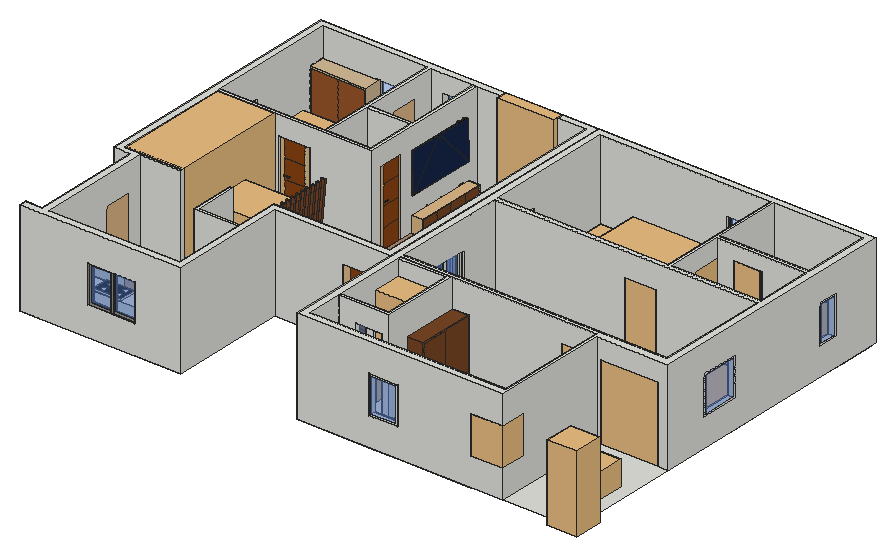
# SketchUp Ruby script. Lengths in inches.
U = 1.inch
M = Sketchup.active_model
def pt(a) = Geom::Point3d.new(a.map { |v| v * U })
def face(e, loops, mat)
  f = e.add_face(loops[0].map { |a| pt(a) })
  loops[1..].each { |l| e.add_face(l.map { |a| pt(a) }).erase! }
  f.material = f.back_material = mat if mat
  f
end
# faces: each face lists its corners as indices into pts; further lists are holes
def faces(e, pts, list, mat = nil) = list.each { |f| face(e, (f[0].is_a?(Array) ? f : [f]).map { |l| l.map { |i| pts[i] } }, mat) }
# xy, xz, yz: faces in a plane at the given z, y or x. An outline is a flat list of corners, or four numbers for a rectangle; further outlines are holes
def ring(l) = l.size == 4 ? [[l[0], l[1]], [l[2], l[1]], [l[2], l[3]], [l[0], l[3]]] : l.each_slice(2).to_a
def flat(e, list, mat, &to3) = list.each { |f| face(e, (f[0].is_a?(Array) ? f : [f]).map { |l| ring(l).map { |u, v| to3.(u, v) } }, mat) }
def xy(e, z, list, mat = nil) = flat(e, list, mat) { |x, y| [x, y, z] }
def xz(e, y, list, mat = nil) = flat(e, list, mat) { |x, z| [x, y, z] }
def yz(e, x, list, mat = nil) = flat(e, list, mat) { |y, z| [x, y, z] }
def lines(e, pts, list) = list.each { |a, b| e.add_line(pt(pts[a]), pt(pts[b])) }
# prism: a flat outline (further loops are holes) pulled along v
def prism(e, loops, v, mat = nil)
  f = face(e, loops, mat); d = Geom::Vector3d.new(v.map { |x| x * U })
  f.pushpull(f.normal.samedirection?(d) ? d.length : -d.length)
end
def box(e, o, s, mat = nil) = prism(e, [[o, [o[0] + s[0], o[1], o[2]], [o[0] + s[0], o[1] + s[1], o[2]], [o[0], o[1] + s[1], o[2]]]], [0, 0, s[2]], mat)
def at(x, y, z, deg = 0) = Geom::Transformation.translation(pt([x, y, z])) * Geom::Transformation.rotation(ORIGIN, Z_AXIS, deg.degrees)
def axes(o, x, y, z) = Geom::Transformation.new([*x, 0, *y, 0, *z, 0, *pt(o).to_a, 1])
def part(name) = M.definitions.add(name)
# library, detail: a bought-in or finely detailed component or shape, given as its bounding box
def library(name, o, s) = part(name).tap { |d| box(d.entities, o, s) }
def detail(e, o, s) = box(e.add_group.entities, o, s)
def put(e, d, t, mat = nil) = e.add_instance(d, t).tap { |i| i.material = mat if mat }
def group(e, t, mat = nil) = e.add_group.tap { |g| g.transformation = t; g.material = mat if mat }.entities
root = M.entities
M.materials.add("Sumele_Jewelry").color = [169, 169, 169]
M.materials.add("Walt_Disney_Pictures_intro_2006").color = [23, 39, 73]
M.materials.add("[0036_BurlyWood]").color = [222, 184, 135]
M.materials.add("[0042_Sienna]").color = [160, 82, 45]
M.materials.add("[0043_SaddleBrown]").color = [139, 69, 19]
M.materials.add("[0136_Charcoal]1").color = [35, 35, 35]
M.materials.add("[0137_Black]").color = [0, 0, 0]
M.materials.add("[Color M03]").color = [170, 170, 170]
M.materials.add("[Color M04]").color = [142, 142, 142]
M.materials.add("[Formica Beige]").color = [211, 187, 149]
M.materials.add("[Tile Veriegated Stone]").color = [171, 137, 112]
M.materials.add("[Translucent Glass Blue]").color = [100, 149, 237]
M.materials["[Translucent Glass Blue]"].alpha = 0.5
M.materials.add("[Wood Cherry Original]").color = [152, 86, 42]
M.materials.add("[Wood Veneer 01]").color = [120, 70, 37]
c1 = library("finestra due ante",[0,0,0],[4.72,47.24,55.51])
c2 = part("Janela aluminio")
xy(c2.entities,0,[[0,0,47.24,1.57],[23.62,1.57,47.24,2.76],[0,2.76,25.98,3.9375],[0,3.9375,47.24,5.91]])
xy(c2.entities,43.31,[[0,0,47.24,1.57],[23.62,1.57,47.24,2.76],[0,2.76,0,5.91,47.24,5.91,47.24,3.9375,25.98,3.9375,25.98,2.76],[25.98,2.76,47.24,3.9375]])
xz(c2.entities,1.57,[[0,0,23.62,0,23.62,41.34,21.26,41.34,21.26,1.97,1.97,1.97,1.97,41.34,23.62,41.34,23.62,43.31,0,43.31],[[23.62,0,47.24,43.31],[25.7,1.97,45.28,41.34]]])
xz(c2.entities,2.76,[[[0,0,23.62,43.31],[2.36,2.36,21.26,40.94]],[23.62,0,25.98,43.31]])
xz(c2.entities,2.76,[[2.36,2.36,21.26,40.94]],"[Translucent Glass Blue]")
xz(c2.entities,3.9375,[[25.98,0,25.98,2.36,44.88,2.36,44.88,40.94,25.98,40.94,25.98,43.31,47.24,43.31,47.24,0]])
xz(c2.entities,3.9375,[[25.98,2.36,44.88,40.94]],"[Translucent Glass Blue]")
yz(c2.entities,0,[[0,0,1.57,43.31],[2.76,0,5.91,43.31]])
yz(c2.entities,23.62,[[1.57,0,2.76,43.31]])
yz(c2.entities,25.98,[[2.76,0,3.9375,43.31]])
yz(c2.entities,47.24,[[0,0,1.57,43.31],[1.57,0,2.76,43.31],[3.9375,0,5.91,43.31]])
c3 = library("Dining Table",[-4.14,-4.14,0],[95.74,137.21,49.0625])
c4 = library("sofa2 (2)",[-0.48,-0.6,0],[71.59,32.48,33.44])
c5 = library("Sofa S1 (2)",[1.47,3.82,0],[91.78,124.8,36.68])
c6 = library("Спалня Венид",[0.07,-0.07,0],[84.71,86.8,39])
c7 = library("70s+Toilet",[-10,-32.21,0],[19.64,32.21,33.59])
c8 = library("60rd,27rd x30h",[0,0,0],[60,60,30.5])
c9 = library("Dressing Table",[-15.16,-2.63,-1.96],[42.78,16.8,62.56])
c10 = library("Shower area",[0,0,0],[40.02,56.82,78.19])
c11 = library("Object02",[-606.68,-655.71,-190.21],[1149.33,653.61,1636.06])
c12 = part("skp42")
put(c12.entities,c11,at(0,0,0))
c13 = part("Senza")
put(c13.entities,c12,at(-166.13,607.08,194.25))
c14 = library("porta 4",[0.2,-5.42,1.33],[46.55,4.72,83.21])
c15 = library("door58",[0,0,0],[34.0625,4.69,78.29])
c16 = library("Vented interior door",[-3.9375,-3.9375,0],[8.49,35.4375,80.68])
c17 = library("Table And Chair",[-36.07,-19.67,0],[55.74,39.34,31.28])
c18 = library("Maple - Red Upright",[-19.73,-16.92,0],[37.29,36.93,96.9])
c19 = library("steps",[5.95,0,1.76],[152,98,97.5])
c20 = library("Sans titre",[-0.34,-1.41,0],[30.55,15.68,32.3])
c21 = part("Group\#3")
xy(c21.entities,0,[[0,1,48,10]])
xy(c21.entities,44.2,[[35,10,46,12]],"[0137_Black]")
xy(c21.entities,45.2,[[35,10,46,12]],"[0137_Black]")
xy(c21.entities,48.93,[[7.7,0,16.7,1]],"[0137_Black]")
xy(c21.entities,49.93,[[7.7,0,16.7,1]],"[0137_Black]")
xy(c21.entities,89,[[0,1,48,10]],"[0036_BurlyWood]")
xz(c21.entities,0,[[7.7,48.93,16.7,49.93]],"[0137_Black]")
xz(c21.entities,1,[[0,0,9.13,0,9.13,48.93,7.7,48.93,7.7,49.93,9.13,49.93,9.13,89,0,89],[40.3,0,48,89]],"[0036_BurlyWood]")
xz(c21.entities,1,[[9.13,0,40.3,22.78],[9.13,22.78,40.3,45.5625],[9.13,45.5625,40.3,45.5625,40.3,68.35,9.13,68.35,9.13,49.93,16.7,49.93,16.7,48.93,9.13,48.93],[9.13,68.35,40.3,89]],"[0043_SaddleBrown]")
xz(c21.entities,10,[[[0,0,48,89],[35,44.2,46,45.2]]],"[0036_BurlyWood]")
xz(c21.entities,12,[[35,44.2,46,45.2]],"[0137_Black]")
yz(c21.entities,0,[[1,0,10,89]],"[0036_BurlyWood]")
yz(c21.entities,7.7,[[0,48.93,1,49.93]],"[0137_Black]")
yz(c21.entities,16.7,[[0,48.93,1,49.93]],"[0137_Black]")
yz(c21.entities,35,[[10,44.2,12,45.2]],"[0137_Black]")
yz(c21.entities,46,[[10,44.2,12,45.2]],"[0137_Black]")
yz(c21.entities,48,[[1,0,10,89]],"[0036_BurlyWood]")
c22 = library("Group\#41",[0,0,0],[50.5,52.39,66.5])
c23 = library("Group\#65",[-3.51,-3.3,0],[107.56,127.46,42.43])
c24 = library("Group\#64",[0,0,0.08],[17.41,128.86,87.4])
c25 = library("组\#105",[-65.55,-8.17,-53.72],[35.57,34.93,21.52])
c26 = library("组\#276",[0,0,0],[31.5,32.28,31.05])
xy(root,16.749,[[351,11.292,351,96.867,360,96.867,360,20.292,442.282,20.292,442.282,11.292],[442.282,11.292,478.282,20.292],[478.282,11.292,571.5,20.292],[571.5,15.792,571.5,20.292,607.5,20.292,607.5,44.292,612,44.292,612,15.792],[607.5,44.292,607.5,164.292,603,164.292,603,168.792,616.5,168.792,616.5,159.792,612,159.792,612,44.292],
  [351,96.867,360,120.818],[351,120.818,351,216.792,360,216.792,360,168.792,564,168.792,564,164.292,360,164.292,360,120.818],[688.5,159.792,688.5,168.792,693,168.792,693,216.792,702,216.792,702,159.792],[351,216.792,360,264.792],[693,216.792,702,264.792],
  [351,264.792,351,328.131,360,328.131,360,317.292,525,317.292,525,312.792,360,312.792,360,264.792],[693,264.792,693,312.792,564,312.792,564,317.292,576,317.292,576,353.292,580.5,353.292,580.5,317.292,693,317.292,693,389.292,634.5,389.292,634.5,393.792,693,393.792,693,400.358,702,400.358,702,264.792],[351,328.131,360,376.131],[351,376.131,351,488.292,520.31,488.292,520.31,479.292,360,479.292,360,376.131],[576,389.292,576,479.292,580.5,479.292,580.5,393.792,601.5,393.792,601.5,389.292],
  [693,400.358,702,424.319],[693,424.319,693,479.292,568.31,479.292,568.31,488.292,702,488.292,702,424.319],[520.31,479.292,568.31,488.292]])
xy(root,16.749,[[0,11.292,15.884,20.292],[[21.884,11.292,204,11.292,204,159.792,351,162.4375,351,488.292,21.884,488.292],[188.5,238.792,193,240.792],[188.5,230.792,193,232.792],[188.5,222.792,193,224.792],[188.5,214.792,193,216.792],[188.5,206.792,193,208.792],[188.5,198.792,193,200.792],[188.5,190.792,193,192.792],[188.5,182.792,193,184.792],[188.5,174.792,193,176.792]],[0,159.792,15.884,488.292]],"[Tile Veriegated Stone]")
xy(root,16.749,[[188.5,174.792,193,176.792],[188.5,182.792,193,184.792],[188.5,190.792,193,192.792],[188.5,198.792,193,200.792],[188.5,206.792,193,208.792],
  [188.5,214.792,193,216.792],[188.5,222.792,193,224.792],[188.5,230.792,193,232.792],[188.5,238.792,193,240.792]],"[Wood Veneer 01]")
xy(root,52.749,[[442.282,11.292,478.282,20.292],[571.5,11.292,612,11.292,612,44.292,607.5,44.292,607.5,20.292,571.5,20.292],[351,96.867,360,120.818],[351,216.792,360,264.792],[693,216.792,702,264.792],
  [351,328.131,360,376.131],[693,400.358,702,424.319],[520.31,479.292,568.31,488.292]])
xy(root,54.656,[[399.065,317.292,512.065,318.292]],"[0137_Black]")
xy(root,59.632,[[204,375.393,206,460.393]],"[0137_Black]")
xy(root,64.749,[[83.903,21.989,119.903,44.041]])
xy(root,64.923,[[140,441.855,141,449.855]],"[0137_Black]")
xy(root,66.749,[[93.688,24.547,94.474,24.65,95.205,24.95,95.834,25.428,96.316,26.051,96.619,26.776,96.722,27.554,96.619,28.333,96.316,29.058,95.834,29.681,95.205,30.158,94.474,30.459,93.688,30.561,92.903,30.459,92.171,30.158,91.543,29.681,91.061,29.058,90.758,28.333,90.654,27.554,90.758,26.776,91.061,26.051,91.543,25.428,92.171,24.95,92.903,24.65],[112.904,24.547,113.689,24.65,114.421,24.95,115.049,25.428,115.531,26.051,115.834,26.776,115.9375,27.554,115.834,28.333,115.531,29.058,115.049,29.681,114.421,30.158,113.689,30.459,112.904,30.561,112.118,30.459,111.387,30.158,110.758,29.681,110.276,29.058,109.973,28.333,109.87,27.554,109.973,26.776,110.276,26.051,110.758,25.428,111.387,24.95,112.118,24.65],[93.688,34.571,94.474,34.673,95.205,34.974,95.834,35.451,96.316,36.074,96.619,36.8,96.722,37.578,96.619,38.356,96.316,39.081,95.834,39.704,95.205,40.182,94.474,40.482,93.688,40.585,92.903,40.482,92.171,40.182,91.543,39.704,91.061,39.081,90.758,38.356,90.654,37.578,90.758,36.8,91.061,36.074,91.543,35.451,92.171,34.974,92.903,34.673],[112.904,34.571,113.689,34.673,114.421,34.974,115.049,35.451,115.531,36.074,115.834,36.8,115.9375,37.578,115.834,38.356,115.531,39.081,115.049,39.704,114.421,40.182,113.689,40.482,112.904,40.585,112.118,40.482,111.387,40.182,110.758,39.704,110.276,39.081,109.973,38.356,109.87,37.578,109.973,36.8,110.276,36.074,110.758,35.451,111.387,34.974,112.118,34.673]])
xy(root,66.749,[[[83.903,21.989,119.903,44.041],[112.904,34.571,112.118,34.673,111.387,34.974,110.758,35.451,110.276,36.074,109.973,36.8,109.87,37.578,109.973,38.356,110.276,39.081,110.758,39.704,111.387,40.182,112.118,40.482,112.904,40.585,113.689,40.482,114.421,40.182,115.049,39.704,115.531,39.081,115.834,38.356,115.9375,37.578,115.834,36.8,115.531,36.074,115.049,35.451,114.421,34.974,113.689,34.673],[93.688,34.571,92.903,34.673,92.171,34.974,91.543,35.451,91.061,36.074,90.758,36.8,90.654,37.578,90.758,38.356,91.061,39.081,91.543,39.704,92.171,40.182,92.903,40.482,93.688,40.585,94.474,40.482,95.205,40.182,95.834,39.704,96.316,39.081,96.619,38.356,96.722,37.578,96.619,36.8,96.316,36.074,95.834,35.451,95.205,34.974,94.474,34.673],[112.904,24.547,112.118,24.65,111.387,24.95,110.758,25.428,110.276,26.051,109.973,26.776,109.87,27.554,109.973,28.333,110.276,29.058,110.758,29.681,111.387,30.158,112.118,30.459,112.904,30.561,113.689,30.459,114.421,30.158,115.049,29.681,115.531,29.058,115.834,28.333,115.9375,27.554,115.834,26.776,115.531,26.051,115.049,25.428,114.421,24.95,113.689,24.65],[93.688,24.547,92.903,24.65,92.171,24.95,91.543,25.428,91.061,26.051,90.758,26.776,90.654,27.554,90.758,28.333,91.061,29.058,91.543,29.681,92.171,30.158,92.903,30.459,93.688,30.561,94.474,30.459,95.205,30.158,95.834,29.681,96.316,29.058,96.619,28.333,96.722,27.554,96.619,26.776,96.316,26.051,95.834,25.428,95.205,24.95,94.474,24.65]]],"[0137_Black]")
xy(root,66.923,[[140,441.855,141,449.855]],"[0137_Black]")
xy(root,70.854,[[145.5,420.773,146.5,427.773]],"[0137_Black]")
xy(root,72.854,[[145.5,420.773,146.5,427.773]],"[0137_Black]")
xy(root,100.749,[[442.282,11.292,478.282,20.292],[571.5,11.292,612,15.792],[571.5,15.792,571.5,20.292,607.5,20.292,607.5,44.292,612,44.292,612,15.792],[351,96.867,360,120.818],[351,216.792,360,264.792],
  [693,216.792,702,264.792],[351,328.131,360,376.131],[693,400.358,702,424.319],[520.31,479.292,568.31,488.292]])
xy(root,101.656,[[399.065,317.292,512.065,318.292]],"[0137_Black]")
xy(root,105.749,[[525,312.792,564,317.292]])
xy(root,109.749,[[564,164.292,603,168.792]])
xy(root,110.632,[[204,375.393,206,460.393]],"[0137_Black]")
xy(root,112.32,[[616.5,159.792,688.5,168.792]])
xy(root,112.749,[[576,353.292,580.5,389.292]])
xy(root,118.749,[[601.5,389.292,634.5,393.792]])
xy(root,136.749,[[[351,11.292,612,11.292,612,159.792,702,159.792,702,488.292,351,488.292],[360,168.792,693,312.792],[360,20.292,607.5,164.292],[360,317.292,576,479.292],[580.5,393.792,693,479.292],[580.5,317.292,693,389.292]]])
xy(root,136.749,[[199.5,174.792,204,176.792],[199.5,182.792,204,184.792],[199.5,190.792,204,192.792],[199.5,198.792,204,200.792],[199.5,206.792,204,208.792],
  [199.5,214.792,204,216.792],[199.5,222.792,204,224.792],[199.5,230.792,204,232.792],[199.5,238.792,204,240.792]],"[Wood Veneer 01]")
xz(root,11.292,[[[351,16.749,612,16.749,612,52.749,571.5,52.749,571.5,100.749,612,100.749,612,136.749,351,136.749],[442.282,52.749,478.282,100.749]],[[442.282,52.749,478.282,100.749],[444.461,54.927,476.103,98.57]]])
xz(root,11.292,[[444.461,54.927,476.103,98.57]],"[Translucent Glass Blue]")
xz(root,20.292,[[[360,16.749,360,136.749,607.5,136.749,607.5,100.749,571.5,100.749,571.5,52.749,607.5,52.749,607.5,16.749],[442.282,52.749,478.282,100.749]]])
xz(root,21.989,[[83.903,64.749,119.903,66.749]])
xz(root,44.041,[[83.903,64.749,119.903,66.749]])
xz(root,44.292,[[607.5,52.749,612,100.749]])
xz(root,96.867,[[351,52.749,360,100.749]])
xz(root,120.818,[[351,52.749,360,100.749]])
xz(root,159.792,[[612,16.749,616.5,16.749,616.5,112.32,688.5,112.32,688.5,16.749,702,16.749,702,136.749,612,136.749]])
xz(root,164.292,[[360,16.749,564,16.749,564,109.749,603,109.749,603,16.749,607.5,16.749,607.5,136.749,360,136.749]])
xz(root,168.792,[[360,16.749,360,136.749,693,136.749,693,16.749,688.5,16.749,688.5,112.32,616.5,112.32,616.5,16.749,603,16.749,603,109.749,564,109.749,564,16.749]])
xz(root,174.792,[[188.5,16.749,193,16.749,204,136.749,199.5,136.749]],"[Wood Veneer 01]")
xz(root,176.792,[[188.5,16.749,199.5,136.749,204,136.749,193,16.749]],"[Wood Veneer 01]")
xz(root,182.792,[[188.5,16.749,193,16.749,204,136.749,199.5,136.749]],"[Wood Veneer 01]")
xz(root,184.792,[[188.5,16.749,199.5,136.749,204,136.749,193,16.749]],"[Wood Veneer 01]")
xz(root,190.792,[[188.5,16.749,193,16.749,204,136.749,199.5,136.749]],"[Wood Veneer 01]")
xz(root,192.792,[[188.5,16.749,199.5,136.749,204,136.749,193,16.749]],"[Wood Veneer 01]")
xz(root,198.792,[[188.5,16.749,193,16.749,204,136.749,199.5,136.749]],"[Wood Veneer 01]")
xz(root,200.792,[[188.5,16.749,199.5,136.749,204,136.749,193,16.749]],"[Wood Veneer 01]")
xz(root,206.792,[[188.5,16.749,193,16.749,204,136.749,199.5,136.749]],"[Wood Veneer 01]")
xz(root,208.792,[[188.5,16.749,199.5,136.749,204,136.749,193,16.749]],"[Wood Veneer 01]")
xz(root,214.792,[[188.5,16.749,193,16.749,204,136.749,199.5,136.749]],"[Wood Veneer 01]")
xz(root,216.792,[[351,52.749,360,100.749],[693,52.749,702,100.749]])
xz(root,216.792,[[188.5,16.749,199.5,136.749,204,136.749,193,16.749]],"[Wood Veneer 01]")
xz(root,222.792,[[188.5,16.749,193,16.749,204,136.749,199.5,136.749]],"[Wood Veneer 01]")
xz(root,224.792,[[188.5,16.749,199.5,136.749,204,136.749,193,16.749]],"[Wood Veneer 01]")
xz(root,230.792,[[188.5,16.749,193,16.749,204,136.749,199.5,136.749]],"[Wood Veneer 01]")
xz(root,232.792,[[188.5,16.749,199.5,136.749,204,136.749,193,16.749]],"[Wood Veneer 01]")
xz(root,238.792,[[188.5,16.749,193,16.749,204,136.749,199.5,136.749]],"[Wood Veneer 01]")
xz(root,240.792,[[188.5,16.749,199.5,136.749,204,136.749,193,16.749]],"[Wood Veneer 01]")
xz(root,264.792,[[351,52.749,360,100.749],[693,52.749,702,100.749]])
xz(root,312.792,[[360,16.749,525,16.749,525,105.749,564,105.749,564,16.749,693,16.749,693,136.749,360,136.749]])
xz(root,317.292,[[[360,16.749,360,136.749,576,136.749,576,16.749,564,16.749,564,105.749,525,105.749,525,16.749],[399.065,54.656,512.065,101.656]],[580.5,16.749,693,136.749]])
xz(root,318.292,[[399.065,54.656,512.065,101.656]],"[0137_Black]")
xz(root,328.131,[[351,52.749,360,100.749]])
xz(root,353.292,[[576,16.749,580.5,112.749]])
xz(root,375.393,[[204,59.632,206,110.632]],"[0137_Black]")
xz(root,376.131,[[351,52.749,360,100.749]])
xz(root,389.292,[[576,16.749,601.5,16.749,601.5,118.749,634.5,118.749,634.5,16.749,693,16.749,693,136.749,580.5,136.749,580.5,112.749,576,112.749]])
xz(root,393.792,[[580.5,16.749,580.5,136.749,693,136.749,693,16.749,634.5,16.749,634.5,118.749,601.5,118.749,601.5,16.749]])
xz(root,400.358,[[693,52.749,702,100.749]])
xz(root,420.773,[[145.5,70.854,146.5,72.854]],"[0137_Black]")
xz(root,424.319,[[693,52.749,702,100.749]])
xz(root,427.773,[[145.5,70.854,146.5,72.854]],"[0137_Black]")
xz(root,441.855,[[140,64.923,141,66.923]],"[0137_Black]")
xz(root,449.855,[[140,64.923,141,66.923]],"[0137_Black]")
xz(root,460.393,[[204,59.632,206,110.632]],"[0137_Black]")
xz(root,479.292,[[[360,16.749,576,136.749],[520.31,52.749,568.31,100.749]],[580.5,16.749,693,136.749]])
xz(root,488.292,[[[351,16.749,702,136.749],[520.31,52.749,568.31,100.749]]])
xz(root,488.292,[[[160.596,84.749,184.557,114.749],[162.026,86.179,183.127,113.319]]],"[Color M04]")
xz(root,488.292,[[162.026,86.179,183.127,113.319]],"[Translucent Glass Blue]")
yz(root,83.903,[[21.989,64.749,44.041,66.749]])
yz(root,119.903,[[21.989,64.749,44.041,66.749]])
yz(root,140,[[441.855,64.923,449.855,66.923]],"[0137_Black]")
yz(root,141,[[441.855,64.923,449.855,66.923]])
yz(root,145.5,[[420.773,70.854,427.773,72.854]])
yz(root,146.5,[[420.773,70.854,427.773,72.854]],"[0137_Black]")
yz(root,204,[[375.393,59.632,460.393,110.632]])
yz(root,206,[[375.393,59.632,460.393,110.632]],"[0137_Black]")
yz(root,351,[[[11.292,16.749,488.292,136.749],[328.131,52.749,376.131,100.749],[216.792,52.749,264.792,100.749],[96.867,52.749,120.818,100.749]],[[96.867,52.749,120.818,100.749],[98.43,54.312,119.255,99.185]]])
yz(root,351,[[98.43,54.312,119.255,99.185]],"[Translucent Glass Blue]")
yz(root,360,[[[20.292,16.749,164.292,136.749],[96.867,52.749,120.818,100.749]],[[168.792,16.749,312.792,136.749],[216.792,52.749,264.792,100.749]],[[317.292,16.749,479.292,136.749],[328.131,52.749,376.131,100.749]]])
yz(root,399.065,[[317.292,54.656,318.292,101.656]],"[0137_Black]")
yz(root,442.282,[[11.292,52.749,20.292,100.749]])
yz(root,478.282,[[11.292,52.749,20.292,100.749]])
yz(root,512.065,[[317.292,54.656,318.292,101.656]])
yz(root,520.31,[[479.292,52.749,488.292,100.749]])
yz(root,525,[[312.792,16.749,317.292,105.749]])
yz(root,564,[[164.292,16.749,168.792,109.749],[312.792,16.749,317.292,105.749]])
yz(root,568.31,[[479.292,52.749,488.292,100.749]])
yz(root,571.5,[[11.292,52.749,20.292,100.749]])
yz(root,576,[[317.292,16.749,317.292,136.749,479.292,136.749,479.292,16.749,389.292,16.749,389.292,112.749,353.292,112.749,353.292,16.749]])
yz(root,580.5,[[317.292,16.749,353.292,16.749,353.292,112.749,389.292,112.749,389.292,136.749,317.292,136.749],[393.792,16.749,479.292,136.749]])
yz(root,601.5,[[389.292,16.749,393.792,118.749]])
yz(root,603,[[164.292,16.749,168.792,109.749]])
yz(root,607.5,[[20.292,16.749,20.292,52.749,44.292,52.749,44.292,100.749,20.292,100.749,20.292,136.749,164.292,136.749,164.292,16.749]])
yz(root,612,[[11.292,16.749,159.792,16.749,159.792,136.749,11.292,136.749,11.292,100.749,44.292,100.749,44.292,52.749,11.292,52.749]])
yz(root,616.5,[[159.792,16.749,168.792,112.32]])
yz(root,634.5,[[389.292,16.749,393.792,118.749]])
yz(root,688.5,[[159.792,16.749,168.792,112.32]])
yz(root,693,[[[168.792,16.749,312.792,136.749],[216.792,52.749,264.792,100.749]],[317.292,16.749,389.292,136.749],[[393.792,16.749,479.292,136.749],[400.358,52.749,424.319,100.749]]])
yz(root,702,[[[159.792,16.749,488.292,136.749],[216.792,52.749,264.792,100.749],[400.358,52.749,424.319,100.749]],[[216.792,52.749,264.792,100.749],[218.515,54.472,263.068,99.026]],[[400.358,52.749,424.319,100.749],[401.857,54.248,422.82,99.249]]])
yz(root,702,[[401.857,54.248,422.82,99.249],[218.515,54.472,263.068,99.026]],"[Translucent Glass Blue]")
p = [[188.5,176.792,16.749],[188.5,174.792,16.749],[199.5,174.792,136.749],[199.5,176.792,136.749],[193,174.792,16.749],[193,176.792,16.749],
  [204,176.792,136.749],[204,174.792,136.749],[188.5,184.792,16.749],[188.5,182.792,16.749],[199.5,182.792,136.749],[199.5,184.792,136.749],
  [193,182.792,16.749],[193,184.792,16.749],[204,184.792,136.749],[204,182.792,136.749],[188.5,192.792,16.749],[188.5,190.792,16.749],
  [199.5,190.792,136.749],[199.5,192.792,136.749],[193,190.792,16.749],[193,192.792,16.749],[204,192.792,136.749],[204,190.792,136.749],
  [188.5,200.792,16.749],[188.5,198.792,16.749],[199.5,198.792,136.749],[199.5,200.792,136.749],[193,198.792,16.749],[193,200.792,16.749],
  [204,200.792,136.749],[204,198.792,136.749],[188.5,208.792,16.749],[188.5,206.792,16.749],[199.5,206.792,136.749],[199.5,208.792,136.749],
  [193,206.792,16.749],[193,208.792,16.749],[204,208.792,136.749],[204,206.792,136.749],[188.5,216.792,16.749],[188.5,214.792,16.749],
  [199.5,214.792,136.749],[199.5,216.792,136.749],[193,214.792,16.749],[193,216.792,16.749],[204,216.792,136.749],[204,214.792,136.749],
  [188.5,224.792,16.749],[188.5,222.792,16.749],[199.5,222.792,136.749],[199.5,224.792,136.749],[193,222.792,16.749],[193,224.792,16.749],
  [204,224.792,136.749],[204,222.792,136.749],[188.5,232.792,16.749],[188.5,230.792,16.749],[199.5,230.792,136.749],[199.5,232.792,136.749],
  [193,230.792,16.749],[193,232.792,16.749],[204,232.792,136.749],[204,230.792,136.749],[188.5,240.792,16.749],[188.5,238.792,16.749],
  [199.5,238.792,136.749],[199.5,240.792,136.749],[193,238.792,16.749],[193,240.792,16.749],[204,240.792,136.749],[204,238.792,136.749],
  [176.053,595.868,20.741],[176.047,595.868,20.73],[176.047,595.86,20.731],[176.053,595.86,20.743],[176.042,595.868,20.717],[176.042,595.86,20.719],
  [176.039,595.868,20.705],[176.039,595.86,20.707],[176.038,595.867,20.692],[176.038,595.859,20.694],[176.06,595.868,20.752],[176.06,595.86,20.754],
  [176.142,595.862,20.793],[176.129,595.863,20.792],[176.129,595.855,20.793],[176.142,595.854,20.795],[176.116,595.865,20.788],[176.115,595.856,20.79],
  [176.103,595.866,20.784],[176.103,595.857,20.786],[176.091,595.866,20.778],[176.091,595.858,20.78],[176.08,595.867,20.77],[176.079,595.859,20.772],
  [176.069,595.868,20.762],[176.069,595.86,20.763],[206.7,592.847,21.003],[206.696,592.849,21.029],[206.696,592.841,21.031],[206.7,592.839,21.005],
  [206.692,592.85,21.041],[206.692,592.842,21.043],[206.685,592.851,21.053],[206.685,592.843,21.055],[206.646,592.857,21.089],[206.634,592.859,21.095],
  [206.634,592.85,21.097],[206.646,592.849,21.091],[206.658,592.855,21.082],[206.658,592.847,21.084],[206.668,592.854,21.073],[206.668,592.846,21.075],
  [206.678,592.853,21.064],[206.677,592.844,21.065],[206.621,592.86,21.099],[206.621,592.852,21.101],[206.594,592.863,21.102],[206.594,592.855,21.104],
  [207.162,416.467,110.119],[206.778,376.199,61.152],[206.774,376.06,61.15],[206,375.515,109.627],[207.223,418.592,110.145],[209.149,459.699,62.065],
  [209.151,459.7,61.968],[208.374,459.153,110.632],[571.5,15.792,16.749],[571.5,15.792,52.749],[206.878,591.971,4.552],[206.878,591.963,4.554],
  [176.216,594.991,4.241],[176.216,594.983,4.242]]
faces(root,p,[[0,1,2,3],[4,5,6,7],[8,9,10,11],[12,13,14,15],[16,17,18,19],[20,21,22,23],[24,25,26,27],[28,29,30,31],
  [32,33,34,35],[36,37,38,39],[40,41,42,43],[44,45,46,47],[48,49,50,51],[52,53,54,55],[56,57,58,59],[60,61,62,63],
  [64,65,66,67],[68,69,70,71]],"[Wood Veneer 01]")
faces(root,p,[[72,73,74,75],[73,76,77,74],[76,78,79,77],[78,80,81,79],[82,72,75,83],[84,85,86,87],[85,88,89,86],[88,90,91,89],
  [90,92,93,91],[92,94,95,93],[94,96,97,95],[96,82,83,97],[98,99,100,101],[99,102,103,100],[102,104,105,103],[106,107,108,109],
  [110,106,109,111],[112,110,111,113],[104,114,115,105],[114,112,113,115],[107,116,117,108],[116,118,119,117]],"[0136_Charcoal]1")
faces(root,p,[[120,121,122,123],[121,120,124,125,126],[125,124,127]],"Walt_Disney_Pictures_intro_2006")
lines(root,p,[[128,129],[130,131],[132,133]])
put(root,c1,axes([306,474.12,16.75],[0,3,0],[-1.524,0,0],[0,0,2.16]),"[Color M03]")
put(root,c2,axes([78,482.39,52.75],[1.016,0,0],[0,1,0],[0,0,1.11]),"[Color M03]")
put(root,c2,axes([345.09,435.87,52.75],[0,-1.016,0],[1,0,0],[0,0,1.10836]),"[Color M03]")
put(root,c2,axes([345.09,264.79,52.75],[0,-1.016,0],[1,0,0],[0,0,1.10836]),"[Color M03]")
put(root,c2,axes([5.91,328.13,52.75],[0,1.016,0],[-1,0,0],[0,0,1.11]))
put(root,c2,axes([5.91,216.79,52.75],[0,1.016,0],[-1,0,0],[0,0,1.11]))
put(root,c2,axes([146,17.2,52.75],[-1.27,0,0],[0,-1,0],[0,0,1.11]),"[Color M04]")
put(root,c3,axes([144.17,210.31,33.1],[0,0.6083,0],[-0.64,0,0],[0,0,1]))
put(root,c4,at(339,218.6,16.75,90))
put(root,c5,axes([339.79,362.67,16.75],[-0.6162,0,0],[0,0.70389,0],[0,0,1]))
put(root,c6,at(94.64,363.1,16.75,90))
put(root,c7,at(145.46,363.1,16.75,90))
put(root,c7,axes([198.65,467.05,16.75],[0,1,0],[1,0,0],[0,0,1]))
put(root,c8,axes([257.42,234.92,16.75],[0.5832,0,0],[0,0.5658,0],[0,0,0.6422]))
put(root,c2,axes([356.91,216.79,52.75],[0,1.016,0],[-1,0,0],[0,0,1.11]))
put(root,c2,axes([356.91,328.13,52.75],[0,1.016,0],[-1,0,0],[0,0,1.11]))
put(root,c2,axes([520.31,482.39,52.75],[1.016,0,0],[0,1,0],[0,0,1.11]),"[Color M03]")
put(root,c9,at(676.68,371.23,28.66,-90))
put(root,c10,axes([630.64,437.3125,15.51],[1.76,0,0],[0,0.8,0],[0,0,0.79]))
put(root,c13,axes([612.74,453.4375,6.65],[0.03254,-0.00139,0],[0.00164,0.03861,0],[0,0,0.02748]))
put(root,c9,axes([373.35,50.88,18.71],[0,-1,0],[-1,0,0],[0,0,1]))
put(root,c14,axes([616.1875,158.46,15.16],[1.54677,0,0],[0,-1.90786,0],[0,0,1.14928]))
put(root,c15,axes([525,312.79,17.86],[1.14493,0,0],[0,1,0],[0,0,1.12251]))
put(root,c16,axes([578.09,357.29,16.75],[0.53001,0,0],[0,1.016,0],[0,0,1.18993]))
put(root,c16,axes([633.5,391.25,16.75],[0,0.49863,0],[-1.016,0,0],[0,0,1.2643]))
put(root,c5,axes([693.8125,222.24,15.74],[-0.6162,0,0],[0,0.70389,0],[0,0,1]))
put(root,c15,axes([564,168.79,16.75],[1.14493,0,0],[0,-1,0],[0,0,1.18784]))
put(root,c10,axes([405.46,123.54,16.75],[0,1.01816,0],[-0.808,0,0],[0,0,1.2877]))
put(root,c7,at(363.63,91.39,20.95,90))
put(root,c17,at(666.25,84.74,16.75))
put(root,c18,at(697.375,15.59,16.73))
put(root,c19,axes([9,318.52,14.59],[0,-0.96217,0],[0.73469,0,0],[0,0,1.23077]))
put(root,c20,at(159.21,316.73,16.75,90))
put(root,c20,at(159.21,384.73,16.75,90))
put(root,c21,at(289.5,158.79,16.75))
g1 = group(root,at(87,312.79,16.75))
xy(g1,0,[[0,0.375,39,3.75]])
xy(g1,47.68,[[28.44,3.75,37.37,4.5]],"[0137_Black]")
xy(g1,48.76,[[28.44,3.75,37.37,4.5]],"[0137_Black]")
xy(g1,52.78,[[6.25,0,13.57,0.375]],"[0137_Black]")
xy(g1,53.86,[[6.25,0,13.57,0.375]],"[0137_Black]")
xy(g1,96,[[0,0.375,39,3.75]],"[0036_BurlyWood]")
xz(g1,0,[[6.25,52.78,13.57,53.86]],"[0137_Black]")
xz(g1,0.375,[[0,0,7.42,0,7.42,52.78,6.25,52.78,6.25,53.86,7.42,53.86,7.42,96,0,96],[32.74,0,39,96]],"[0036_BurlyWood]")
xz(g1,0.375,[[7.42,0,32.74,24.57],[7.42,24.57,32.74,49.15],[7.42,49.15,32.74,49.15,32.74,73.73,7.42,73.73,7.42,53.86,13.57,53.86,13.57,52.78,7.42,52.78],[7.42,73.73,32.74,96]],"[0043_SaddleBrown]")
xz(g1,3.75,[[[0,0,39,96],[28.44,47.68,37.37,48.76]]],"[0036_BurlyWood]")
xz(g1,4.5,[[28.44,47.68,37.37,48.76]],"[0137_Black]")
yz(g1,0,[[0.375,0,3.75,96]],"[0036_BurlyWood]")
yz(g1,6.25,[[0,52.78,0.375,53.86]],"[0137_Black]")
yz(g1,13.57,[[0,52.78,0.375,53.86]],"[0137_Black]")
yz(g1,28.44,[[3.75,47.68,4.5,48.76]],"[0137_Black]")
yz(g1,37.37,[[3.75,47.68,4.5,48.76]],"[0137_Black]")
yz(g1,39,[[0.375,0,3.75,96]],"[0036_BurlyWood]")
put(root,c21,axes([204.23,326.29,16.75],[0,0.6875,0],[-0.39417,0,0],[0,0,1.07865]))
g2 = group(root,at(0,11.29,16.75))
xy(g2,0,[[0,0,0,9,21,9,21,100.5,30,100.5,30,9,86,9,86,0],[146,0,146,9,195,9,195,157.5,289.5,157.5,289.5,148.5,204,148.5,204,0],[21,133.5,21,148.5,0,148.5,0,205.5,9,205.5,9,157.5,81,157.5,81,153,30,153,30,133.5],[337.5,148.5,337.5,157.5,342,157.5,342,205.5,351,205.5,351,148.5],[0,205.5,9,253.5],
  [342,205.5,351,253.5],[0,253.5,9,316.84],[342,253.5,351,376.58],[9,301.5,87,306],[126,301.5,126,306,199.5,306,199.5,315,204,315,204,301.5],
  [141,306,145.5,408],[0,316.84,9,364.84],[199.5,348,199.5,367.5,145.5,367.5,145.5,372,199.5,372,199.5,468,204,468,204,348],[0,364.84,0,477,78,477,78,468,9,468,9,364.84],[342,376.58,351,424.58],
  [342,424.58,342,468,306,468,306,477,351,477,351,424.58],[141,441,145.5,468],[78,468,126,477],[126,468,160.6,477],[160.6,468,184.56,477],
  [184.56,468,234,477]])
xy(g2,36,[[86,0,146,9],[0,205.5,9,253.5],[342,205.5,351,253.5],[0,316.84,9,364.84],[342,376.58,351,424.58],
  [78,468,126,477]])
xy(g2,68,[[160.6,468,184.56,477]])
xy(g2,84,[[86,0,146,9],[21,100.5,30,133.5],[0,205.5,9,253.5],[342,205.5,351,253.5],[0,316.84,9,364.84],
  [342,376.58,351,424.58],[78,468,126,477]])
xy(g2,89,[[289.5,148.5,337.5,157.5]])
xy(g2,96,[[87,301.5,126,306],[199.5,315,204,348],[141,408,145.5,441]])
xy(g2,98,[[160.6,468,184.56,477]])
xy(g2,120,[[0,0,204,0,204,148.5,351,148.5,351,477,306,477,306,468,342,468,342,157.5,195,157.5,195,9,30,9,30,153,81,153,81,157.5,9,157.5,9,468,141,468,141,306,145.5,306,145.5,468,234,468,234,477,0,477,0,148.5,21,148.5,21,9,0,9],[9,301.5,204,301.5,204,468,199.5,468,199.5,372,145.5,372,145.5,367.5,199.5,367.5,199.5,306,9,306]])
xz(g2,0,[[[0,0,204,120],[86,36,146,84]]])
xz(g2,9,[[0,0,21,120],[[30,0,195,120],[86,36,146,84]]])
xz(g2,100.5,[[21,0,30,84]])
xz(g2,133.5,[[21,0,30,84]])
xz(g2,148.5,[[0,0,21,120],[204,0,289.5,0,289.5,89,337.5,89,337.5,0,351,0,351,120,204,120]])
xz(g2,153,[[30,0,81,120]])
xz(g2,157.5,[[9,0,81,120],[195,0,195,120,342,120,342,0,337.5,0,337.5,89,289.5,89,289.5,0]])
xz(g2,205.5,[[0,36,9,84],[342,36,351,84]])
xz(g2,253.5,[[0,36,9,84],[342,36,351,84]])
xz(g2,301.5,[[9,0,87,0,87,96,126,96,126,0,204,0,204,120,9,120]])
xz(g2,306,[[9,0,9,120,141,120,141,0,126,0,126,96,87,96,87,0],[141,0,145.5,120],[145.5,0,199.5,120]])
xz(g2,315,[[199.5,0,204,96]])
xz(g2,316.84,[[0,36,9,84]])
xz(g2,348,[[199.5,0,204,96]])
xz(g2,364.84,[[0,36,9,84]])
xz(g2,367.5,[[145.5,0,199.5,120]])
xz(g2,372,[[145.5,0,199.5,120]])
xz(g2,376.58,[[342,36,351,84]])
xz(g2,408,[[141,0,145.5,96]])
xz(g2,424.58,[[342,36,351,84]])
xz(g2,441,[[141,0,145.5,96]])
xz(g2,468,[[[9,0,141,120],[78,36,126,84]],[[145.5,0,199.5,120],[160.6,68,184.56,98]],[199.5,0,204,120],[204,0,234,120],[306,0,342,120]])
xz(g2,477,[[[0,0,234,120],[78,36,126,84],[160.6,68,184.56,98]],[306,0,351,120]])
yz(g2,0,[[0,0,9,120],[[148.5,0,477,120],[316.84,36,364.84,84],[205.5,36,253.5,84]]])
yz(g2,9,[[[157.5,0,301.5,120],[205.5,36,253.5,84]],[301.5,0,306,120],[[306,0,468,120],[316.84,36,364.84,84]]])
yz(g2,21,[[9,0,9,120,148.5,120,148.5,0,133.5,0,133.5,84,100.5,84,100.5,0]])
yz(g2,30,[[9,0,100.5,0,100.5,84,133.5,84,133.5,0,153,0,153,120,9,120]])
yz(g2,78,[[468,36,477,84]])
yz(g2,81,[[153,0,157.5,120]])
yz(g2,86,[[0,36,9,84]])
yz(g2,87,[[301.5,0,306,96]])
yz(g2,126,[[301.5,0,306,96],[468,36,477,84]])
yz(g2,141,[[306,0,306,120,468,120,468,0,441,0,441,96,408,96,408,0]])
yz(g2,145.5,[[306,0,367.5,120],[367.5,0,372,120],[372,0,408,0,408,96,441,96,441,0,468,0,468,120,372,120]])
yz(g2,146,[[0,36,9,84]])
yz(g2,160.6,[[468,68,477,98]])
yz(g2,184.56,[[468,68,477,98]])
yz(g2,195,[[9,0,157.5,120]])
yz(g2,199.5,[[306,0,306,120,367.5,120,367.5,0,348,0,348,96,315,96,315,0],[372,0,468,120]])
yz(g2,204,[[0,0,148.5,120],[301.5,0,315,0,315,96,348,96,348,0,468,0,468,120,301.5,120]])
yz(g2,234,[[468,0,477,120]])
yz(g2,289.5,[[148.5,0,157.5,89]])
yz(g2,306,[[468,0,477,120]])
yz(g2,337.5,[[148.5,0,157.5,89]])
yz(g2,342,[[[157.5,0,468,120],[376.58,36,424.58,84],[205.5,36,253.5,84]]])
yz(g2,351,[[[148.5,0,477,120],[376.58,36,424.58,84],[205.5,36,253.5,84]]])
g3 = group(root,at(141,419.29,16.75),"[0137_Black]")
xy(g3,0,[[0,0,4.5,33]])
xy(g3,96,[[0,0,4.5,33]],"[0036_BurlyWood]")
xz(g3,0,[[0,0,4.5,96]],"[0036_BurlyWood]")
xz(g3,33,[[0,0,4.5,96]],"[0036_BurlyWood]")
yz(g3,0,[[0,0,0,43.8,30.36,0],[33,0,0,48,33,96],[0,51.84,0,96,30.36,96]],"[0036_BurlyWood]")
yz(g3,0,[[30.36,0,0,43.8,0,48,33,0],[0,48,0,51.84,30.36,96,33,96]],"[0042_Sienna]")
yz(g3,4.5,[[0,0,33,96]],"[0036_BurlyWood]")
put(root,c21,axes([21,144.79,16.75],[0,-0.6875,0],[0.91667,0,0],[0,0,0.94382]))
g4 = group(root,at(139.5,111.79,16.75))
prism(g4,[[[0,0,0],[0,57,0],[4.5,57,0],[4.5,4.5,0],[55.5,4.5,0],[55.5,0,0]]],[0,0,120])
g5 = group(root,at(30,20.29,16.75))
prism(g5,[[[0,0,0],[0,91.5,0],[21,91.5,0],[21,24,0],[165,24,0],[165,0,0]]],[0,0,48])
g6 = group(root,at(9,458.29,16.75))
xy(g6,0,[[0,0,72,21]])
xy(g6,84,[[0,0,72,21]],"[Formica Beige]")
xz(g6,0,[[[0,0,72,84],[1.69,1.69,70.31,82.31]]],"[Formica Beige]")
xz(g6,0,[[1.69,1.69,36,82.31],[36,1.69,70.31,82.31]],"[Wood Cherry Original]")
xz(g6,21,[[0,0,72,84]])
yz(g6,0,[[0,0,21,84]])
yz(g6,72,[[0,0,21,84]],"[Formica Beige]")
g7 = group(root,at(81,458.29,16.75))
box(g7,[0,0,0],[60,21,24])
g8 = group(root,at(204,375.15,16.75),"[0036_BurlyWood]")
xy(g8,0,[[0,0,15,90]])
xy(g8,20,[[0,0,15,90]])
xz(g8,0,[[0,0,15,20]])
xz(g8,90,[[0,0,15,20]])
yz(g8,0,[[0,0,90,20]])
yz(g8,15,[[[0,0,90,20],[0.71,0.71,89.29,19.29]]],"[0036_BurlyWood]")
yz(g8,15,[[0.71,0.71,22.85,19.29],[22.85,0.71,45,19.29],[45,0.71,67.15,19.29],[67.15,0.71,89.29,19.29]],"[Wood Veneer 01]")
g9 = group(root,at(176.37,80.32,16.75))
xy(g9,0,[[1,0,17.62,27]])
xy(g9,23.65,[[0,23.32,1,24.32]],"[0137_Black]")
xy(g9,35.65,[[0,23.32,1,24.32]],"[0137_Black]")
xy(g9,41,[[1,0,17.62,27]])
xy(g9,42.67,[[0,23.38,1,24.38]],"[0137_Black]")
xy(g9,48.67,[[0,23.38,1,24.38]],"[0137_Black]")
xy(g9,54,[[1,0,17.62,27]])
xz(g9,0,[[1,0,17.62,41],[1,41,17.62,54]])
xz(g9,23.32,[[0,23.65,1,35.65]],"[0137_Black]")
xz(g9,23.38,[[0,42.67,1,48.67]],"[0137_Black]")
xz(g9,24.32,[[0,23.65,1,35.65]],"[0137_Black]")
xz(g9,24.38,[[0,42.67,1,48.67]],"[0137_Black]")
xz(g9,27,[[1,0,17.62,41],[1,41,17.62,54]])
yz(g9,0,[[23.32,23.65,24.32,35.65],[23.38,42.67,24.38,48.67]],"[0137_Black]")
yz(g9,1,[[[0,0,27,41],[23.32,23.65,24.32,35.65]],[[0,41,27,54],[23.38,42.67,24.38,48.67]]])
yz(g9,17.62,[[0,0,27,41],[0,41,27,54]])
put(root,c22,axes([571.5,45.79,52.75],[0.80198,0,0],[0,-0.6585,0],[0,0,0.7218]))
g10 = group(root,at(580.5,317.29,16.75))
xy(g10,0,[[0,0,112.5,24]])
xy(g10,2.15,[[2.15,2,110.35,24]])
xy(g10,86.85,[[2.15,2,110.35,24]])
xy(g10,89,[[0,0,112.5,24]],"Sumele_Jewelry")
xz(g10,0,[[0,0,112.5,89]],"Sumele_Jewelry")
xz(g10,2,[[2.15,2.15,110.35,86.85]])
xz(g10,24,[[[0,0,112.5,89],[2.15,2.15,110.35,86.85]],[56.25,2.15,2.15,44.5,2.15,51.48,56.25,10.14],[56.25,2.15,56.25,10.14,110.35,60.21,110.35,54.42]])
xz(g10,24,[[2.15,2.15,2.15,44.5,56.25,2.15],[56.25,2.15,110.35,54.42,110.35,2.15],[56.25,10.14,2.15,51.48,2.15,86.85,56.25,86.85],[56.25,10.14,56.25,86.85,110.35,86.85,110.35,60.21]],"Sumele_Jewelry")
yz(g10,0,[[0,0,24,89]],"Sumele_Jewelry")
yz(g10,2.15,[[2,2.15,24,86.85]])
yz(g10,110.35,[[2,2.15,24,86.85]])
yz(g10,112.5,[[0,0,24,89]],"Sumele_Jewelry")
put(root,c23,axes([501.34,476.14,16.65],[0,-0.9,0],[-0.8,0,0],[0,0,1]))
put(root,c24,axes([571.91,13.68,16.71],[0,1,0],[-0.74427,0,0],[0,0,1]))
g11 = group(root,at(424.5,92.29,16.75),"[Wood Veneer 01]")
xy(g11,0,[[0,0,21,72]])
xy(g11,84,[[0,0,21,72]])
xz(g11,0,[[0,0,21,84]])
xz(g11,72,[[0,0,21,84]])
yz(g11,0,[[0,0,72,84]])
yz(g11,21,[[[0,0,72,84],[1.0625,1.0625,70.9375,82.9375]],[1.0625,1.0625,36,82.9375],[36,1.0625,70.9375,82.9375]])
put(root,c23,axes([580.21,35.31,16.65],[0,0.9,0],[-0.8,0,0],[0,0,1]))
put(root,c25,at(389.93,506.28,70.57,90))
put(root,c26,axes([390.23,353.9,16.85],[0,-0.9801,0],[-0.88209,0,0],[0,0,0.9801]))
put(root,c26,axes([390.23,429.9,16.85],[0,-0.9801,0],[-0.88209,0,0],[0,0,0.9801]))
g12 = group(root,at(351,11.29,16.75))
xy(g12,0,[[0,0,351,477]])
g13 = group(root,at(360,65.29,16.75))
xy(g13,0,[[0,0,22.5,4.5],[55.5,0,55.5,4.5,60,4.5,60,94.5,0,94.5,0,99,64.5,99,64.5,0]])
xy(g13,96,[[22.5,0,55.5,4.5]])
xy(g13,120,[[0,0,64.5,0,64.5,99,0,99,0,94.5,60,94.5,60,4.5,0,4.5]])
xz(g13,0,[[0,0,22.5,0,22.5,96,55.5,96,55.5,0,64.5,0,64.5,120,0,120]])
xz(g13,4.5,[[0,0,0,120,60,120,60,96,22.5,96,22.5,0],[55.5,0,60,96]])
xz(g13,94.5,[[0,0,60,120]])
xz(g13,99,[[0,0,64.5,120]])
yz(g13,0,[[0,0,4.5,120],[94.5,0,99,120]])
yz(g13,22.5,[[0,0,4.5,96]])
yz(g13,55.5,[[0,0,4.5,96]])
yz(g13,60,[[4.5,0,94.5,120]])
yz(g13,64.5,[[0,0,99,120]])
